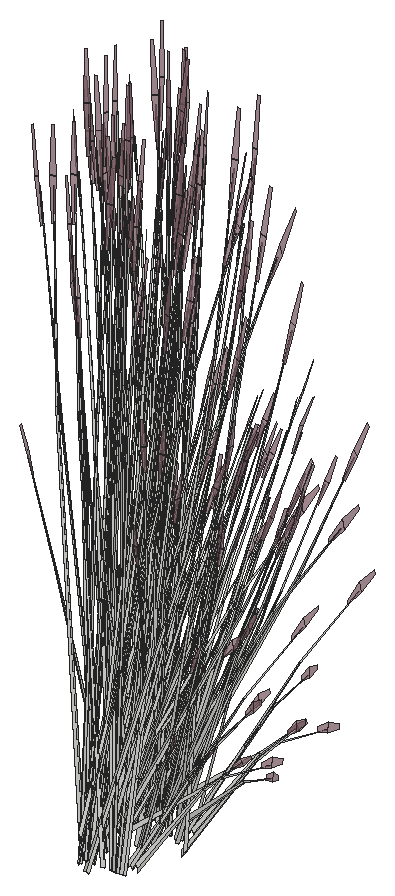
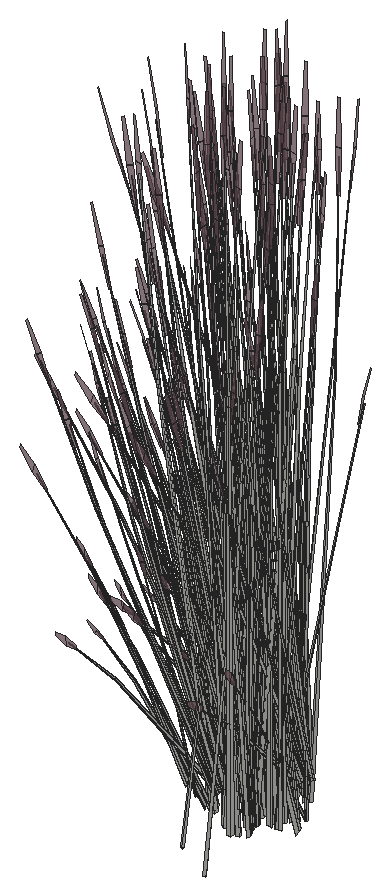
# SketchUp Ruby script. Lengths in inches.
U = 1.inch
M = Sketchup.active_model
def pt(a) = Geom::Point3d.new(a.map { |v| v * U })
def face(e, loops, mat)
  f = e.add_face(loops[0].map { |a| pt(a) })
  loops[1..].each { |l| e.add_face(l.map { |a| pt(a) }).erase! }
  f.material = f.back_material = mat if mat
  f
end
# faces: each face lists its corners as indices into pts; further lists are holes
def faces(e, pts, list, mat = nil) = list.each { |f| face(e, (f[0].is_a?(Array) ? f : [f]).map { |l| l.map { |i| pts[i] } }, mat) }
# xy, xz, yz: faces in a plane at the given z, y or x. An outline is a flat list of corners, or four numbers for a rectangle; further outlines are holes
def ring(l) = l.size == 4 ? [[l[0], l[1]], [l[2], l[1]], [l[2], l[3]], [l[0], l[3]]] : l.each_slice(2).to_a
def flat(e, list, mat, &to3) = list.each { |f| face(e, (f[0].is_a?(Array) ? f : [f]).map { |l| ring(l).map { |u, v| to3.(u, v) } }, mat) }
def xy(e, z, list, mat = nil) = flat(e, list, mat) { |x, y| [x, y, z] }
def xz(e, y, list, mat = nil) = flat(e, list, mat) { |x, z| [x, y, z] }
def yz(e, x, list, mat = nil) = flat(e, list, mat) { |y, z| [x, y, z] }
def lines(e, pts, list) = list.each { |a, b| e.add_line(pt(pts[a]), pt(pts[b])) }
# prism: a flat outline (further loops are holes) pulled along v
def prism(e, loops, v, mat = nil)
  f = face(e, loops, mat); d = Geom::Vector3d.new(v.map { |x| x * U })
  f.pushpull(f.normal.samedirection?(d) ? d.length : -d.length)
end
def box(e, o, s, mat = nil) = prism(e, [[o, [o[0] + s[0], o[1], o[2]], [o[0] + s[0], o[1] + s[1], o[2]], [o[0], o[1] + s[1], o[2]]]], [0, 0, s[2]], mat)
def at(x, y, z, deg = 0) = Geom::Transformation.translation(pt([x, y, z])) * Geom::Transformation.rotation(ORIGIN, Z_AXIS, deg.degrees)
def axes(o, x, y, z) = Geom::Transformation.new([*x, 0, *y, 0, *z, 0, *pt(o).to_a, 1])
def part(name) = M.definitions.add(name)
# library, detail: a bought-in or finely detailed component or shape, given as its bounding box
def library(name, o, s) = part(name).tap { |d| box(d.entities, o, s) }
def detail(e, o, s) = box(e.add_group.entities, o, s)
def put(e, d, t, mat = nil) = e.add_instance(d, t).tap { |i| i.material = mat if mat }
def group(e, t, mat = nil) = e.add_group.tap { |g| g.transformation = t; g.material = mat if mat }.entities
root = M.entities
M.materials.add("LightPink_Translucent").color = [144, 107, 117]
M.materials["LightPink_Translucent"].alpha = 0.75
c1 = part("blade")
p = [[2.15,0.21,22],[0,0.17,0],[0.09,0.45,0],[2.18,0.31,22],[2.29,0.31,22],[0.38,0.45,0],
  [2.48,0.24,33],[2.49,0.24,33],[2.48,0.22,33]]
faces(c1.entities,p,[[0,1,2,3],[4,5,2,3],[6,3,4,7],[8,0,3,6]])
c2 = part("seeds")
p = [[0.3,-0.1,1.38],[-0.01,-0.03,1.59],[-0.01,-0.03,0.03],[0.14,-0.07,-0.07],[0.29,-0.03,3],[0.15,0.01,3.11]]
faces(c2.entities,p,[[0,1,2,3],[1,0,4,5]],"LightPink_Translucent")
c3 = part("blade with seeds")
put(c3.entities,c1,at(0,0,0))
put(c3.entities,c2,axes([2.4,0.25,30.99],[1.5799,-0.05474,1.17369],[-0.12525,1.92788,0.29478],[-0.07173,-0.02425,1.56792]))
put(root,c3,axes([296.16,463.82,2.47],[0.25843,-0.64844,0.17642],[0.9457,0.1835,0.35086],[-0.16336,0.00316,1.60407]))
put(root,c3,axes([297.88,466.03,1.49],[-0.1339,-0.0514,1.76342],[-0.34394,-0.57425,-0.26939],[0.23202,-0.15583,0.30037]))
put(root,c3,axes([295.94,462.35,2.21],[0.62448,0.42144,0],[-0.62448,0.42144,0],[0,0,1.69266]))
put(root,c3,axes([297.63,462.17,2.47],[-0.70288,-0.47526,0.17642],[0.70832,-0.46097,0.35086],[-0.07763,0.09706,1.60407]))
put(root,c3,axes([296.33,461.45,2.06],[0.9306,0.10697,-0.62353],[-0.19638,0.65984,-0.16365],[0.27771,0.07995,1.37633]))
put(root,c3,axes([295.11,466.16,5.05],[-0.2697,0.50175,0.35414],[-0.78684,-0.14635,-0.4572],[-0.07215,-0.20201,0.87481]))
put(root,c3,axes([300.44,462.61,2.77],[-0.55274,0.10771,1.1486],[0.26018,-0.44517,0.84392],[0.29323,0.03046,0.25299]))
put(root,c3,axes([297.125,466.375,4.73],[0.63704,0.44518,0.48003],[-0.67652,0.38394,0.3958],[0.11751,-0.20886,0.9933]))
put(root,c3,axes([294.53,463.89,2.2],[-0.90188,-0.29293,0],[0.43405,-0.60866,0],[0,0,1.62707]))
put(root,c3,axes([297.36,466.42,4.73],[0.73517,0.0304,0.0643],[-0.02016,0.45906,0.50621],[0.07693,-0.17585,0.77189]))
put(root,c3,axes([295.93,461.86,2.72],[0.43405,-0.58792,0.44739],[0.90188,0.28295,-0.21531],[0,0.13553,1.43643]))
put(root,c3,axes([296.81,466.73,5.05],[-0.60531,0.34352,0.35414],[-0.573,-0.39225,-0.4572],[0.08718,-0.19929,0.87481]))
put(root,c3,axes([300.1875,464.49,4.71],[-0.08089,-0.05712,1.77383],[0.17695,-0.61228,-0.16761],[0.31864,-0.03912,0.31391]))
put(root,c3,axes([297.875,467.65,4.98],[0.4673,-0.51481,-0.71045],[0.81887,0.36587,0.08574],[0.27902,-0.18652,1.00501]))
put(root,c3,axes([292.82,466.15,2.375],[-0.55932,-0.6538,0],[0.93577,-0.36461,-0.51607],[0.21313,-0.08304,1.63711]))
put(root,c3,axes([297.85,467.41,4.68],[-0.22982,-0.59576,-0.51099],[0.87033,-0.10422,-0.3958],[0.24941,-0.16002,0.97773]))
put(root,c3,axes([295.77,462.2,2.29],[0,0.75458,-0.05637],[-1.11865,0,0],[0,0.02371,1.79368]))
put(root,c3,axes([295.85,461.66,2.21],[0.53742,0.54764,-0.44739],[-0.81403,0.38564,0.21531],[0.17391,0.06776,1.43643]))
put(root,c3,axes([299.48,463.98,3.93],[-0.17122,-0.54847,-0.03492],[0.80929,-0.12609,-0.15832],[0.169,0.03477,0.52218]))
put(root,c3,axes([297.38,463.96,5.03],[0.0479,-0.66354,-0.1216],[0.90696,0.01814,-0.67495],[0.3493,0.04609,1.02557]))
put(root,c3,axes([298.26,467.84,5.03],[-0.82753,-0.35977,-0.1216],[0.47675,-0.52101,-0.67495],[0.2338,-0.18111,1.02557]))
put(root,c3,axes([298.21,462.1875,2.48],[0,-0.65246,0.49651],[1.00089,0,0],[0,0.1486,1.57504]))
put(root,c3,axes([295.7,462.68,2.72],[0.97146,-0.04028,0.44739],[0.08785,0.66859,-0.21531],[-0.17391,0.06776,1.43643]))
put(root,c3,axes([296.31,462,2.62],[0.83351,-0.19028,0.1448],[0.29189,0.54335,-0.41347],[0,0.11958,1.26744]))
put(root,c3,axes([297.25,463.7,5.05],[-0.50902,-0.40851,0.35414],[0.58122,-0.38671,-0.4572],[0.29531,0.05884,0.87481]))
put(root,c3,axes([299.41,463.32,2.59],[-0.21545,-0.16047,1.43002],[0.28033,-0.53085,-0.30754],[0.43591,0.07191,0.61141]))
put(root,c3,axes([293.58,466.05,2.02],[0.83726,-0.32623,-0.49651],[0.50045,0.58498,0],[0.19069,-0.0743,1.57504]))
put(root,c3,axes([298.55,467.18,2.59],[-0.31959,-0.01933,1.43002],[-0.32741,-0.51843,-0.30754],[0.39262,-0.14666,0.61141]))
put(root,c3,axes([300.3,467.68,4.71],[-0.11685,-0.00496,1.77383],[-0.48522,-0.53096,-0.16761],[0.19486,-0.17458,0.31391]))
put(root,c3,axes([295.56,463.9,2.2],[0.90188,0.29293,0],[-0.43405,0.60866,0],[0,0,1.74954]))
put(root,c3,axes([294.58,467.39,2.06],[0.60257,-0.49041,-0.62353],[0.74854,0.44469,-0.16365],[0.24146,-0.12234,1.37633]))
put(root,c3,axes([298.92,466.23,2.77],[-0.29798,0.33213,1.1486],[-0.25612,-0.44624,0.84392],[0.24611,-0.11182,0.25299]))
put(root,c3,axes([298.17,463.5625,4.72],[0.19191,-0.01103,1.74944],[0.52639,-0.5069,-0.27667],[0.34136,0.06691,0.14031]))
put(root,c3,axes([295.72,462.96,2.62],[0.66093,0.39201,0.1448],[-0.5513,0.44227,-0.41347],[-0.15345,0.05979,1.26744]))
put(root,c3,axes([298.5,467.47,4.53],[0.77872,-0.09325,-0.35414],[0.20563,0.53305,0.4572],[0.22316,-0.14318,0.87481]))
put(root,c3,axes([293.53,468.25,2.21],[0.43405,-0.58792,-0.44739],[0.90188,0.28295,0.21531],[0,-0.13553,1.43643]))
put(root,c3,axes([297.43,463.64,4.98],[0.89428,0.01571,-0.71045],[-0.06006,0.66153,0.08574],[0.37886,0.06981,1.00501]))
put(root,c3,axes([293.92,467.96,2.67],[-0.10425,-0.7445,-0.29095],[1.08575,-0.04502,-0.50002],[0.19119,-0.09917,1.59708]))
put(root,c3,axes([296.42,464.17,2.48],[0.83726,-0.32623,0.49651],[0.50045,0.58498,0],[-0.19069,0.0743,1.57504]))
put(root,c3,axes([297.86,467.79,5.05],[-0.77872,0.09325,0.35414],[-0.20563,-0.53305,-0.4572],[0.22316,-0.14318,0.87481]))
put(root,c3,axes([295.23,463.66,2.29],[0.38895,0.74956,-0.06012],[-1.11135,0.26265,0],[0.01358,0.02618,1.72173]))
put(root,c3,axes([298.89,462.3,2.375],[1.11865,0,0],[0,0.72922,-0.51607],[0,0.16609,1.63711]))
put(root,c3,axes([293.78,466.31,2.03],[0.83462,0.16144,-0.30978],[-0.21015,0.56852,0.30978],[0.16826,-0.06556,1.38974]))
put(root,c3,axes([298.44,462.67,2.2],[-1.1181,-0.00522,-0.04976],[0,-0.72922,0.49943],[-0.03514,0.166,1.58352]))
put(root,c3,axes([296.02,462.04,2.67],[1.00749,0.31132,-0.29095],[-0.48511,0.65709,-0.50002],[0.03166,0.16133,1.59708]))
put(root,c3,axes([297.97,463.92,4.53],[0.50902,0.40851,-0.35414],[-0.58122,0.38671,0.4572],[0.29531,0.05884,0.87481]))
put(root,c3,axes([298.21,462.78,2.03],[-0.62448,0.40708,-0.30978],[-0.62448,-0.40708,0.30978],[0,0.13112,1.38974]))
put(root,c3,axes([297.71,464.07,4.73],[-0.04505,0.49615,0.0643],[-0.68022,-0.0136,0.50621],[0.26056,0.05192,0.77189]))
put(root,c3,axes([295.92,462.53,2.21],[-0.43405,0.58792,-0.44739],[-0.90188,-0.28295,0.21531],[0,0.13553,1.43643]))
put(root,c3,axes([297.77,463.91,4.73],[-0.65964,0.42992,0.48003],[-0.5689,-0.45657,0.3958],[0.30948,0.0793,0.9933]))
put(root,c3,axes([298.57,467.7,4.73],[0.61415,0.2744,0.0643],[-0.35756,0.39076,0.50621],[0.1969,-0.12633,0.77189]))
put(root,c3,axes([298.39,467.59,4.73],[0.22187,0.60049,0.48003],[-0.87033,0.10422,0.3958],[0.25651,-0.14123,0.9933]))
put(root,c3,axes([300.74,468.32,4.72],[0.12414,-0.09938,1.74944],[-0.15889,-0.60963,-0.27667],[0.31148,-0.11559,0.14031]))
put(root,c3,axes([295.67,464.41,5.05],[-0.13817,-0.52554,0.35414],[0.78985,-0.13877,-0.4572],[0.21215,0.1506,0.87481]))
put(root,c3,axes([294.07,468.54,2.43],[1.00799,0.31623,0.24065],[-0.48511,0.65709,0.50002],[0,-0.15147,1.60543]))
put(root,c3,axes([295.9375,464.21,2.33],[1.11998,0.21207,0.30756],[-0.2802,0.75803,-0.36492],[-0.18537,0.09487,1.64885]))
put(root,c3,axes([298.64,462.79,2.02],[0,0.65246,-0.49651],[-1.00089,0,0],[0,0.1486,1.57504]))
put(root,c3,axes([296.14,462.87,3.875],[-0.3323,-0.11241,1.71376],[0.68769,-0.4716,0.13857],[0.42861,0.21275,0.73262]))
put(root,c3,axes([296.2,461.39,4.47],[-0.77304,-0.33901,1.38283],[0.81626,-0.52782,0.59665],[0.24941,0.31809,1.33663]))
put(root,c3,axes([297.37,464.15,2.77],[-0.5037,-0.18761,1.1486],[0.6504,-0.19062,0.84392],[0.17543,0.16147,0.25299]))
put(root,c3,axes([293.74,468.1,2.72],[-0.97146,0.04028,0.44739],[-0.08785,-0.66859,-0.21531],[0.17391,-0.06776,1.43643]))
put(root,c3,axes([295.6,464.68,5.03],[0.53309,-0.55848,-0.1216],[0.77201,0.32175,-0.67495],[0.26836,0.15779,1.02557]))
put(root,c3,axes([298.3,469.24,5.03],[-0.45012,-0.59081,-0.1216],[0.79888,-0.29033,-0.67495],[0.33665,-0.07795,1.02557]))
put(root,c3,axes([298.26,468.73,4.68],[0.24236,-0.59349,-0.51099],[0.83094,0.20343,-0.3958],[0.33455,-0.05442,0.97773]))
put(root,c3,axes([296.94,466.32,2.375],[0.55932,-0.6538,0],[0.93577,0.36461,-0.51607],[0.21313,0.08304,1.63711]))
put(root,c3,axes([293.71,468.34,2.36],[0.38895,0.72959,0.45755],[-1.11135,0.2537,0.17955],[0.01358,-0.13406,1.58856]))
put(root,c3,axes([296.62,464.625,2.375],[0.55932,0.6538,0],[-0.93577,0.36461,-0.51607],[-0.21313,0.08304,1.63711]))
put(root,c3,axes([299.15,468.9,1.98],[-0.57619,0.0783,1.41583],[-0.09171,-0.62326,0.08104],[0.40356,-0.09434,0.80566]))
put(root,c3,axes([300.19,468.35,2.26],[-0.55463,-0.41721,-0.06488],[0.60744,-0.38228,-0.29416],[0.17212,-0.02691,0.97024]))
put(root,c3,axes([294.9,465.15,4.71],[0.00265,-0.07899,1.77383],[0.76665,-0.34851,-0.16761],[0.2663,0.12439,0.31391]))
put(root,c3,axes([297.51,464.84,1.49],[0.06518,-0.0942,1.76342],[0.82057,-0.27742,-0.26939],[0.24877,0.14358,0.30037]))
put(root,c3,axes([296.43,462.71,2.09],[0.32803,0.59738,-0.69212],[-0.94492,0.21515,-0.18165],[0.03626,0.20229,1.52773]))
put(root,c3,axes([295.11,468.4,2.21],[0,-0.75495,0],[1.11865,0,0],[0,0,1.79456]))
put(root,c3,axes([296.23,464.41,4.68],[0.88277,-0.1551,-0.51099],[0.15442,0.58737,-0.3958],[0.23711,0.16832,0.97773]))
put(root,c3,axes([296.46,466.66,2.48],[-0.83726,-0.32623,0.49651],[0.50045,-0.58498,0],[0.19069,0.0743,1.57504]))
put(root,c3,axes([298.1,468.95,4.98],[0.78611,-0.28816,-0.71045],[0.4381,0.59317,0.08574],[0.37982,-0.06738,1.00501]))
put(root,c3,axes([293.78,464.49,5.05],[0.2697,-0.50175,0.35414],[0.78684,0.14635,-0.4572],[0.07215,0.20201,0.87481]))
put(root,c3,axes([294.58,467.93,2.36],[-0.74176,0.59212,0.45755],[-0.88124,-0.52269,0.17955],[0.17882,-0.05909,1.58856]))
put(root,c3,axes([297.45,465,2.67],[-0.57368,-0.02046,1.0506],[0.37886,-0.43461,0.58006],[0.22663,0.15441,0.8241]))
put(root,c3,axes([295.39,468.99,2.3],[-0.83213,-0.56158,-0.06131],[0.83263,-0.56193,0],[-0.02906,-0.01961,1.75571]))
put(root,c3,axes([293.29,466.95,2.47],[-0.25843,0.64844,0.17642],[-0.9457,-0.1835,0.35086],[0.16336,-0.00316,1.60407]))
put(root,c3,axes([297.98,469.0625,5.05],[-0.74348,-0.18202,0.35414],[0.21685,-0.53102,-0.4572],[0.29933,-0.04869,0.87481]))
put(root,c3,axes([295.8,464.89,4.73],[-0.4066,0.41448,0.0643],[-0.57901,-0.24131,0.50621],[0.18719,0.13288,0.77189]))
put(root,c3,axes([292.9,467.48,1.59],[-0.88056,0.26122,1.28929],[-0.28027,-0.74951,0.50096],[0.54072,0.01247,1.46642]))
put(root,c3,axes([294.84,466.28,5.65],[0.61821,-0.37431,-0.06488],[0.56645,0.40995,-0.29416],[0.03988,0.11616,0.97024]))
put(root,c3,axes([295.26,467.67,2.62],[0.17258,-0.58229,0.1448],[0.84319,0.10108,-0.41347],[0.15345,0.05979,1.26744]))
put(root,c3,axes([295.97,464.77,4.73],[-0.88979,0.14973,0.48003],[-0.15442,-0.58737,0.3958],[0.20926,0.17311,0.9933]))
put(root,c3,axes([299.77,468.49,1.49],[-0.04675,-0.09906,1.76342],[0.32428,-0.57943,-0.26939],[0.32711,-0.00833,0.30037]))
put(root,c3,axes([294.9,467.83,2.72],[-0.53742,-0.54764,0.44739],[0.81403,-0.38564,-0.21531],[0.17391,0.06776,1.43643]))
put(root,c3,axes([295.58,463.95,2.59],[0.01579,-0.21629,1.43002],[0.75442,-0.24159,-0.30754],[0.23289,0.25887,0.61141]))
put(root,c3,axes([293.54,464.95,4.73],[-0.6592,0.22175,0.0643],[-0.32265,-0.40436,0.50621],[0.06366,0.17825,0.77189]))
put(root,c3,axes([295.18,467.86,2.67],[0.90324,-0.43318,-0.29095],[0.60064,0.61207,-0.50002],[0.22285,0.06216,1.59708]))
put(root,c3,axes([293.52,464.71,5.03],[0.87543,-0.30377,-0.1216],[0.4302,0.53915,-0.67495],[0.1155,0.2272,1.02557]))
put(root,c3,axes([298.77,469,4.53],[0.74348,0.18202,-0.35414],[-0.21685,0.53102,0.4572],[0.29933,-0.04869,0.87481]))
put(root,c3,axes([293.77,464.91,5.0625],[-0.88151,-0.17057,0.53283],[0.30143,-0.56078,0.43934],[0.05297,0.22053,1.10256]))
put(root,c3,axes([297.45,466.71,2.02],[0.83726,0.32623,-0.49651],[-0.50045,0.58498,0],[0.19069,0.0743,1.57504]))
put(root,c3,axes([295.86,468.57,2.21],[1.00089,0,0],[0,0.67548,0],[0,0,1.78407]))
put(root,c3,axes([293.68,464.82,1.49],[0.14478,-0.0355,1.76342],[0.8709,0.19542,-0.26939],[0.02547,0.22025,0.30037]))
put(root,c3,axes([296.15,466.99,2.47],[-0.96132,0.17317,0.17642],[-0.23737,-0.64447,0.35086],[0.08574,0.0939,1.60407]))
put(root,c3,axes([296.74,468.35,3.875],[-0.37107,0.01478,1.71376],[0.24616,-0.64047,0.13857],[0.5288,0.03961,0.73262]))
put(root,c3,axes([297.22,466.95,2.03],[0.21015,0.56852,-0.30978],[-0.83462,0.16144,0.30978],[0.16826,0.06556,1.38974]))
put(root,c3,axes([294.27,464.68,4.68],[0.87941,0.16356,-0.51099],[-0.30143,0.56078,-0.3958],[0.08064,0.22578,0.97773]))
put(root,c3,axes([298.66,469.23,4.73],[0.32857,0.44488,0.0643],[-0.59916,0.21775,0.50621],[0.26412,-0.04296,0.77189]))
put(root,c3,axes([294.77,463.52,3.875],[-0.2045,-0.20949,1.71376],[0.94495,-0.17636,0.13857],[0.21357,0.32887,0.73262]))
put(root,c3,axes([295.54,468.23,2.38],[-1.13071,-0.13747,0.49198],[0.23011,-0.77639,0.19306],[0.16524,0.07497,1.70813]))
put(root,c3,axes([298.59,469.07,4.73],[-0.25275,0.59491,0.48003],[-0.83094,-0.20343,0.3958],[0.32677,-0.03575,0.9933]))
put(root,c3,axes([294.64,470.15,2.2],[-0.29189,-0.56252,0],[0.83351,-0.19699,0],[0,0,1.54371]))
put(root,c3,axes([293.87,465.02,4.53],[-0.2697,0.50175,-0.35414],[-0.78684,-0.14635,0.4572],[0.07215,0.20201,0.87481]))
put(root,c3,axes([295.73,470.07,2.18],[0.93921,-0.22138,-0.19198],[0.33003,0.6377,0.00008],[0.10367,-0.02447,1.73897]))
put(root,c3,axes([296.06,470.33,2.47],[0.25843,-0.64844,0.17642],[0.9457,0.1835,0.35086],[-0.16336,0.00316,1.60407]))
put(root,c3,axes([295.84,468.86,2.21],[0.62448,0.42144,0],[-0.62448,0.42144,0],[0,0,1.69266]))
put(root,c3,axes([297.53,468.68,2.47],[-0.70288,-0.47526,0.17642],[0.70832,-0.46097,0.35086],[-0.07763,0.09706,1.60407]))
put(root,c3,axes([296.23,467.96,2.06],[0.9306,0.10697,-0.62353],[-0.19638,0.65984,-0.16365],[0.27771,0.07995,1.37633]))
put(root,c3,axes([300.34,469.11,2.77],[-0.55274,0.10771,1.1486],[0.26018,-0.44517,0.84392],[0.29323,0.03046,0.25299]))
put(root,c3,axes([295.83,468.37,2.72],[0.43405,-0.58792,0.44739],[0.90188,0.28295,-0.21531],[0,0.13553,1.43643]))
put(root,c3,axes([293.95,464.57,4.98],[0.42698,0.53052,-0.71045],[-0.87893,0.29566,0.08574],[0.09984,0.25633,1.00501]))
put(root,c3,axes([300.09,471,4.71],[-0.08089,-0.05712,1.77383],[0.17695,-0.61228,-0.16761],[0.31864,-0.03912,0.31391]))
put(root,c3,axes([295.67,468.7,2.29],[0,0.75458,-0.05637],[-1.11865,0,0],[0,0.02371,1.79368]))
put(root,c3,axes([295.75,468.17,2.21],[0.53742,0.54764,-0.44739],[-0.81403,0.38564,0.21531],[0.17391,0.06776,1.43643]))
put(root,c3,axes([293.3125,465.91,4.72],[0.1134,0.10507,1.74944],[0.91515,0.04128,-0.27667],[0.09203,0.23172,0.14031]))
put(root,c3,axes([299.38,470.49,3.93],[-0.17122,-0.54847,-0.03492],[0.80929,-0.12609,-0.15832],[0.169,0.03477,0.52218]))
put(root,c3,axes([297.29,470.47,5.03],[0.0479,-0.66354,-0.1216],[0.90696,0.01814,-0.67495],[0.3493,0.04609,1.02557]))
put(root,c3,axes([298.11,468.7,2.48],[0,-0.65246,0.49651],[1.00089,0,0],[0,0.1486,1.57504]))
put(root,c3,axes([295.6,469.18,2.72],[0.97146,-0.04028,0.44739],[0.08785,0.66859,-0.21531],[-0.17391,0.06776,1.43643]))
put(root,c3,axes([296.21,468.5,2.62],[0.83351,-0.19028,0.1448],[0.29189,0.54335,-0.41347],[0,0.11958,1.26744]))
put(root,c3,axes([297.15,470.21,5.05],[-0.50902,-0.40851,0.35414],[0.58122,-0.38671,-0.4572],[0.29531,0.05884,0.87481]))
put(root,c3,axes([299.31,469.83,2.59],[-0.21545,-0.16047,1.43002],[0.28033,-0.53085,-0.30754],[0.43591,0.07191,0.61141]))
put(root,c3,axes([295.46,470.41,2.2],[0.90188,0.29293,0],[-0.43405,0.60866,0],[0,0,1.74954]))
put(root,c3,axes([298.07,470.07,4.72],[0.19191,-0.01103,1.74944],[0.52639,-0.5069,-0.27667],[0.34136,0.06691,0.14031]))
put(root,c3,axes([295.62,469.47,2.62],[0.66093,0.39201,0.1448],[-0.5513,0.44227,-0.41347],[-0.15345,0.05979,1.26744]))
put(root,c3,axes([297.33,470.15,4.98],[0.89428,0.01571,-0.71045],[-0.06006,0.66153,0.08574],[0.37886,0.06981,1.00501]))
put(root,c3,axes([296.32,470.68,2.48],[0.83726,-0.32623,0.49651],[0.50045,0.58498,0],[-0.19069,0.0743,1.57504]))
put(root,c3,axes([295.13,470.16,2.29],[0.38895,0.74956,-0.06012],[-1.11135,0.26265,0],[0.01358,0.02618,1.72173]))
put(root,c3,axes([298.79,468.81,2.375],[1.11865,0,0],[0,0.72922,-0.51607],[0,0.16609,1.63711]))
put(root,c3,axes([298.34,469.18,2.2],[-1.1181,-0.00522,-0.04976],[0,-0.72922,0.49943],[-0.03514,0.166,1.58352]))
put(root,c3,axes([295.93,468.55,2.67],[1.00749,0.31132,-0.29095],[-0.48511,0.65709,-0.50002],[0.03166,0.16133,1.59708]))
put(root,c3,axes([297.87,470.42,4.53],[0.50902,0.40851,-0.35414],[-0.58122,0.38671,0.4572],[0.29531,0.05884,0.87481]))
put(root,c3,axes([298.11,469.29,2.03],[-0.62448,0.40708,-0.30978],[-0.62448,-0.40708,0.30978],[0,0.13112,1.38974]))
put(root,c3,axes([297.61,470.58,4.73],[-0.04505,0.49615,0.0643],[-0.68022,-0.0136,0.50621],[0.26056,0.05192,0.77189]))
put(root,c3,axes([295.82,469.04,2.21],[-0.43405,0.58792,-0.44739],[-0.90188,-0.28295,0.21531],[0,0.13553,1.43643]))
put(root,c3,axes([293.55,477.4,2.59],[-0.25429,0.13207,1.43002],[-0.76157,-0.23115,-0.30754],[0.14117,-0.28747,0.61141]))
put(root,c3,axes([297.67,470.42,4.73],[-0.65964,0.42992,0.48003],[-0.5689,-0.45657,0.3958],[0.30948,0.0793,0.9933]))
put(root,c3,axes([295.57,470.92,5.05],[-0.13817,-0.52554,0.35414],[0.78985,-0.13877,-0.4572],[0.21215,0.1506,0.87481]))
put(root,c3,axes([294.17,478.38,4.98],[0.02328,-0.60353,-0.71045],[0.98022,0.04053,0.08574],[0.10344,-0.25568,1.00501]))
put(root,c3,axes([295.84,470.72,2.33],[1.11998,0.21207,0.30756],[-0.2802,0.75803,-0.36492],[-0.18537,0.09487,1.64885]))
